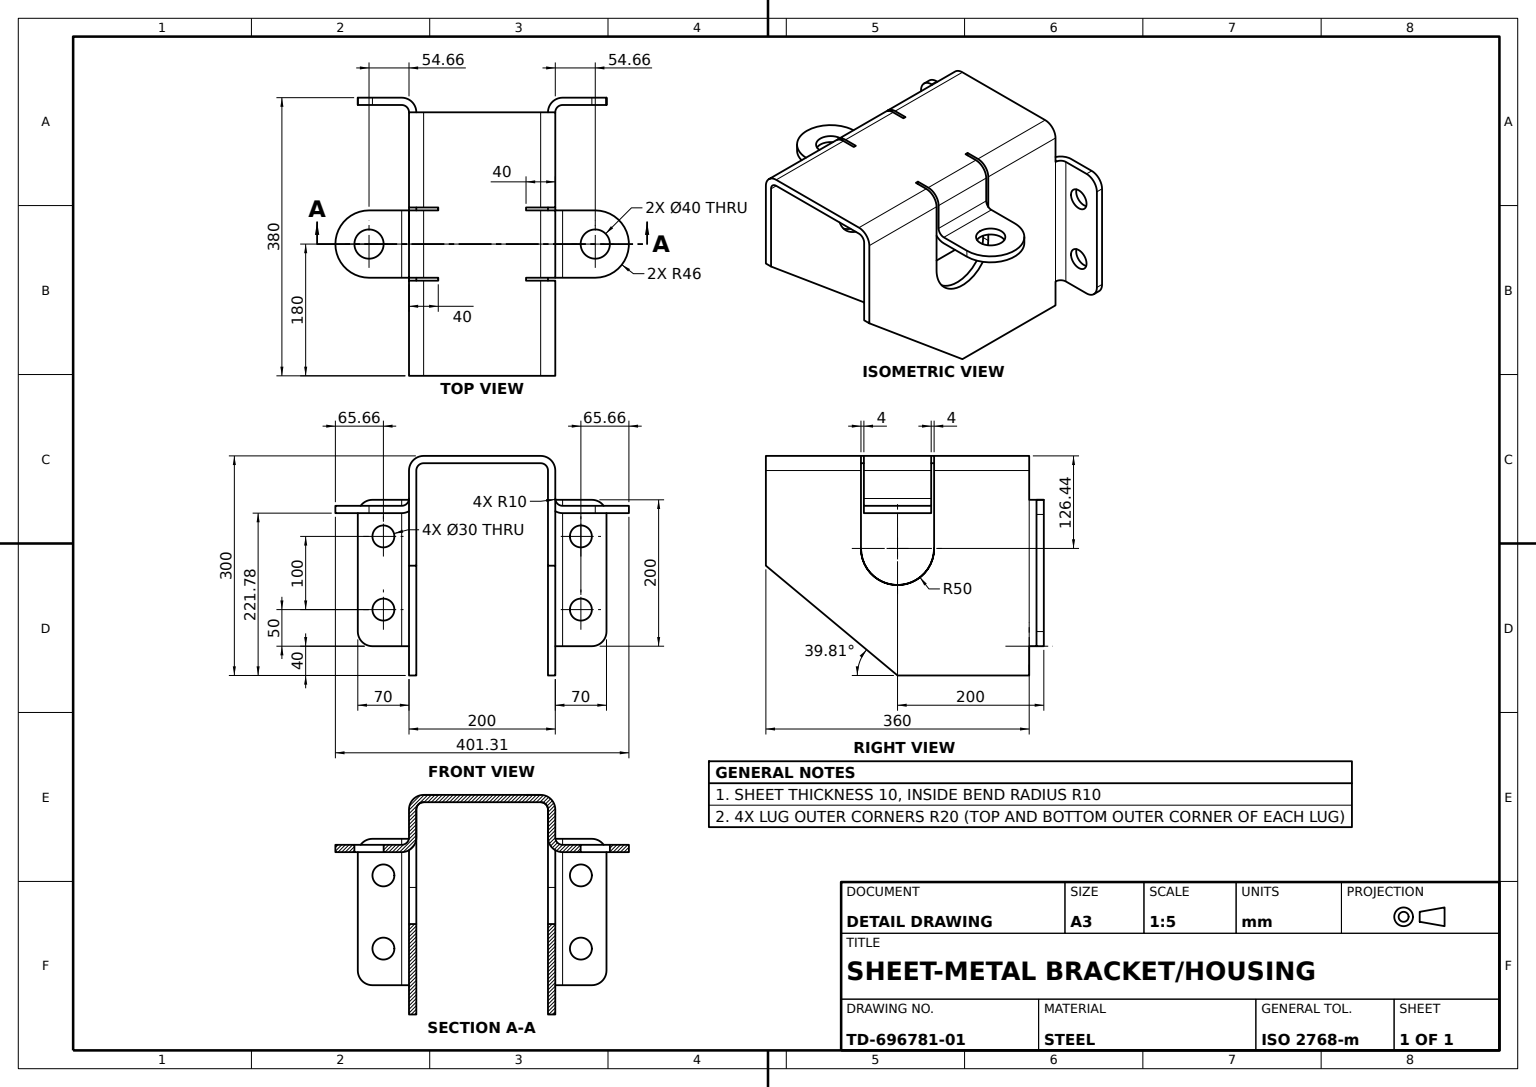
solid
v1 (0,-300,-100)
v2 (0,-300,-90)
e1 v1 v2 LINE
v3 (-180,-300,-90)
e2 v2 v3 LINE
v4 (-180,-300,-100)
e3 v4 v3 LINE
e4 v1 v4 LINE
face PLANE(AX(P(-180,-300,-100),D(0,1,0),D(0,0,1))) rev [e1 e2 -e3 -e4]
v5 (-46,0,-80)
v6 (-46,0,-60)
e5 v5 v6 LINE
v7 (-46,-10,-80)
e6 v7 v5 LINE
v8 (-46,-10,-60)
e7 v7 v8 LINE
e8 v8 v6 LINE
face PLANE(AX(P(-46,-10,-60),D(-1,0,0),D(0,0,1))) [-e5 -e6 e7 e8]
v9 (-46,-78.219028,110)
v10 (-46,-58.219028,90)
e9 v9 v10 CIRCLE(AX(P(-46,-58.219028,110),D(1,0,0),D(0,1,0)),20)
v11 (46,-58.219028,90)
e10 v11 v10 LINE
v12 (46,-78.219028,110)
e11 v11 v12 CIRCLE(AX(P(46,-58.219028,110),D(-1,0,0),D(0,-1,0)),20)
e12 v12 v9 LINE
face CYL(AX(P(95.49432,-58.219028,110),D(-1,0,0),D(0,-1,0)),20) [e9 -e10 e11 e12]
v13 (46,-68.219028,154.657083)
v14 (0,-68.219028,200.657083)
e13 v13 v14 CIRCLE(AX(P(0,-68.219028,154.657083),D(0,-1,0),D(0,0,1)),46)
v15 (0,-78.219028,200.657083)
e14 v15 v14 LINE
v16 (46,-78.219028,154.657083)
e15 v16 v15 CIRCLE(AX(P(0,-78.219028,154.657083),D(0,-1,0),D(0,0,1)),46)
e16 v16 v13 LINE
face CYL(AX(P(0,-78.219028,154.657083),D(0,1,0),D(0,0,1)),46) [e13 -e14 -e15 e16]
v17 (46,-20,-100)
v18 (46,0,-80)
e17 v17 v18 CIRCLE(AX(P(46,-20,-80),D(1,0,0),D(0,0,-1)),20)
v19 (-46,-20,-100)
e18 v19 v17 LINE
e19 v5 v19 CIRCLE(AX(P(-46,-20,-80),D(-1,0,0),D(0,0,-1)),20)
e20 v18 v5 LINE
face CYL(AX(P(-95.49432,-20,-80),D(1,0,0),D(0,0,-1)),20) [-e17 -e18 -e19 -e20]
v20 (-180,-300,100)
v21 (-180,-260,100)
e21 v20 v21 LINE
v22 (0,-300,100)
e22 v22 v20 LINE
v23 (180,-150,100)
e23 v23 v22 LINE
v24 (180,-20,100)
e24 v24 v23 LINE
v25 (50,-20,100)
e25 v24 v25 LINE
v26 (50,-126.438055,100)
e26 v26 v25 LINE
v27 (0,-176.438055,100)
e27 v27 v26 CIRCLE(AX(P(0,-126.438055,100),D(0,0,1),D(0,-1,0)),50)
v28 (-50,-126.438055,100)
e28 v28 v27 CIRCLE(AX(P(0,-126.438055,100),D(0,0,1),D(0,-1,0)),50)
v29 (-50,-20,100)
e29 v29 v28 LINE
v30 (-180,-20,100)
e30 v29 v30 LINE
v31 (-180,-60,100)
e31 v31 v30 LINE
e32 v21 v31 LINE
face PLANE(AX(P(0,0,100),D(0,0,1),D(0,-1,0))) [-e21 -e22 -e23 -e24 e25 -e26 -e27 -e28 -e29 e30 -e31 -e32]
v32 (-180,-60,-100)
v33 (-180,-20,-100)
e33 v32 v33 LINE
v34 (-50,-20,-100)
e34 v33 v34 LINE
v35 (-50,-126.438055,-100)
e35 v34 v35 LINE
v36 (50,-126.438055,-100)
e36 v35 v36 CIRCLE(AX(P(0,-126.438055,-100),D(0,0,1),D(0,-1,0)),50)
v37 (50,-20,-100)
e37 v36 v37 LINE
v38 (180,-20,-100)
e38 v37 v38 LINE
v39 (180,-150,-100)
e39 v38 v39 LINE
e40 v39 v1 LINE
v40 (-180,-260,-100)
e41 v4 v40 LINE
e42 v32 v40 LINE
face PLANE(AX(P(0,0,-100),D(0,0,-1),D(0,-1,0))) [e33 e34 e35 e36 e37 e38 e39 e40 e4 e41 -e42]
v41 (-200,-210,120)
v42 (-200,-210,150)
e43 v41 v42 CIRCLE(AX(P(-200,-210,135),D(-1,0,0),D(0,0,1)),15)
v43 (-190,-210,150)
e44 v42 v43 LINE
v44 (-190,-210,120)
e45 v44 v43 CIRCLE(AX(P(-190,-210,135),D(-1,0,0),D(0,0,1)),15)
e46 v41 v44 LINE
face CYL(AX(P(-200,-210,135),D(1,0,0),D(0,0,-1)),15) rev [e43 e44 -e45 -e46]
v45 (-46,-20,-90)
e47 v19 v45 LINE
e48 v7 v45 CIRCLE(AX(P(-46,-20,-80),D(-1,0,0),D(0,0,-1)),10)
face PLANE(AX(P(-46,-20,-80),D(1,0,0),D(0,0,-1))) rev [e6 e19 e47 -e48]
v46 (46,-20,-90)
v47 (46,-10,-80)
e49 v46 v47 CIRCLE(AX(P(46,-20,-80),D(1,0,0),D(0,0,1)),10)
e50 v47 v7 LINE
e51 v45 v46 LINE
face CYL(AX(P(-95.49432,-20,-80),D(1,0,0),D(0,0,-1)),10) rev [e49 e50 e48 e51]
v48 (46,-10,60)
v49 (46,-10,80)
e52 v48 v49 LINE
v50 (46,0,60)
e53 v48 v50 LINE
v51 (46,0,80)
e54 v50 v51 LINE
e55 v49 v51 LINE
face PLANE(AX(P(46,-10,60),D(-1,0,0),D(0,0,1))) rev [-e52 e53 e54 -e55]
v52 (-190,-60,110)
v53 (-190,-260,110)
e56 v52 v53 LINE
e57 v21 v53 CIRCLE(AX(P(-180,-260,110),D(0,1,0),D(0,0,1)),10)
e58 v52 v31 CIRCLE(AX(P(-180,-60,110),D(0,-1,0),D(0,0,1)),10)
face CYL(AX(P(-180,-361.631261,110),D(0,1,0),D(0,0,1)),10) rev [e56 -e57 e32 -e58]
v54 (46,-58.219028,-100)
e59 v17 v54 LINE
v55 (-46,-58.219028,-100)
e60 v55 v54 LINE
e61 v55 v19 LINE
face PLANE(AX(P(0,0,-100),D(0,0,-1),D(0,-1,0))) [e59 -e60 e61 e18]
v56 (50,-10,80)
v57 (180,-10,80)
e62 v56 v57 LINE
v58 (180,-20,90)
e63 v57 v58 CIRCLE(AX(P(180,-20,80),D(1,0,0),D(0,0,-1)),10)
v59 (50,-20,90)
e64 v58 v59 LINE
e65 v59 v56 CIRCLE(AX(P(50,-20,80),D(-1,0,0),D(0,0,1)),10)
face CYL(AX(P(247.495907,-20,80),D(-1,0,0),D(0,0,1)),10) rev [e62 e63 e64 e65]
v60 (46,-78.219028,-110)
v61 (46,-78.219028,-154.657083)
e66 v60 v61 LINE
v62 (46,-68.219028,-154.657083)
e67 v61 v62 LINE
v63 (46,-68.219028,-110)
e68 v63 v62 LINE
e69 v63 v60 LINE
face PLANE(AX(P(46,-78.219028,-4.657083),D(1,0,0),D(0,0,-1))) [e66 e67 -e68 e69]
v64 (46,-20,100)
e70 v51 v64 CIRCLE(AX(P(46,-20,80),D(1,0,0),D(0,0,1)),20)
v65 (46,-20,90)
e71 v64 v65 LINE
e72 v49 v65 CIRCLE(AX(P(46,-20,80),D(1,0,0),D(0,0,-1)),10)
face PLANE(AX(P(46,-20,80),D(-1,0,0),D(0,0,1))) rev [e70 e71 -e72 e55]
v66 (0,-78.219028,134.657083)
v67 (0,-68.219028,134.657083)
e73 v66 v67 LINE
v68 (0,-78.219028,174.657083)
e74 v68 v66 CIRCLE(AX(P(0,-78.219028,154.657083),D(0,1,0),D(0,0,1)),20)
v69 (0,-68.219028,174.657083)
e75 v68 v69 LINE
e76 v69 v67 CIRCLE(AX(P(0,-68.219028,154.657083),D(0,1,0),D(0,0,1)),20)
face CYL(AX(P(0,-78.219028,154.657083),D(0,1,0),D(0,0,1)),20) rev [-e73 -e74 e75 e76]
v70 (180,-150,90)
e77 v23 v70 LINE
e78 v58 v70 LINE
e79 v58 v24 LINE
face PLANE(AX(P(180,-150,100),D(1,0,0),D(0,1,0))) [e24 e77 -e78 e79]
v71 (180,-10,-80)
v72 (50,-10,-80)
e80 v71 v72 LINE
v73 (50,-20,-90)
e81 v72 v73 CIRCLE(AX(P(50,-20,-80),D(-1,0,0),D(0,0,-1)),10)
v74 (180,-20,-90)
e82 v73 v74 LINE
e83 v74 v71 CIRCLE(AX(P(180,-20,-80),D(1,0,0),D(0,0,-1)),10)
face CYL(AX(P(-17.495907,-20,-80),D(1,0,0),D(0,0,-1)),10) rev [e80 e81 e82 e83]
v75 (-200,-110,150)
v76 (-200,-110,120)
e84 v75 v76 CIRCLE(AX(P(-200,-110,135),D(-1,0,0),D(0,0,1)),15)
v77 (-190,-110,120)
e85 v76 v77 LINE
v78 (-190,-110,150)
e86 v78 v77 CIRCLE(AX(P(-190,-110,135),D(-1,0,0),D(0,0,1)),15)
e87 v75 v78 LINE
face CYL(AX(P(-200,-110,135),D(1,0,0),D(0,0,-1)),15) rev [e84 e85 -e86 -e87]
v79 (-50,-126.438055,-90)
e88 v79 v35 LINE
v80 (50,-126.438055,-90)
e89 v79 v80 CIRCLE(AX(P(0,-126.438055,-90),D(0,0,1),D(0,-1,0)),50)
e90 v80 v36 LINE
face CYL(AX(P(0,-126.438055,-90),D(0,0,-1),D(0,1,0)),50) rev [-e36 -e88 e89 e90]
v81 (-46,-78.219028,-154.657083)
e91 v61 v81 CIRCLE(AX(P(0,-78.219028,-154.657083),D(0,1,0),D(0,0,-1)),46)
v82 (-46,-68.219028,-154.657083)
e92 v81 v82 LINE
e93 v62 v82 CIRCLE(AX(P(0,-68.219028,-154.657083),D(0,1,0),D(0,0,-1)),46)
face CYL(AX(P(0,-78.219028,-154.657083),D(0,1,0),D(0,0,1)),46) [e91 e92 -e93 -e67]
v83 (0,-68.219028,-134.657083)
v84 (0,-68.219028,-174.657083)
e94 v83 v84 CIRCLE(AX(P(0,-68.219028,-154.657083),D(0,-1,0),D(0,0,-1)),20)
v85 (0,-78.219028,-134.657083)
e95 v85 v83 LINE
v86 (0,-78.219028,-174.657083)
e96 v85 v86 CIRCLE(AX(P(0,-78.219028,-154.657083),D(0,-1,0),D(0,0,-1)),20)
e97 v86 v84 LINE
face CYL(AX(P(0,-78.219028,-154.657083),D(0,1,0),D(0,0,1)),20) rev [-e94 -e95 e96 e97]
v87 (-200,-260,110)
e98 v53 v87 LINE
v88 (-190,-260,150)
e99 v53 v88 LINE
v89 (-200,-260,150)
e100 v89 v88 LINE
e101 v87 v89 LINE
face PLANE(AX(P(-200,-260,150),D(0,1,0),D(0,0,1))) rev [-e98 e99 -e100 -e101]
v90 (-46,-68.219028,-110)
e102 v55 v90 CIRCLE(AX(P(-46,-58.219028,-110),D(1,0,0),D(0,0,-1)),10)
v91 (-46,-78.219028,-110)
e103 v91 v90 LINE
v92 (-46,-58.219028,-90)
e104 v92 v91 CIRCLE(AX(P(-46,-58.219028,-110),D(1,0,0),D(0,0,-1)),20)
e105 v92 v55 LINE
face PLANE(AX(P(-46,-58.219028,-110),D(-1,0,0),D(0,0,1))) [e102 -e103 -e104 e105]
v93 (-180,-260,90)
v94 (-180,-60,90)
e106 v93 v94 LINE
e107 v93 v87 CIRCLE(AX(P(-180,-260,110),D(0,1,0),D(-1,0,0)),20)
v95 (-200,-60,110)
e108 v95 v87 LINE
e109 v95 v94 CIRCLE(AX(P(-180,-60,110),D(0,-1,0),D(0,0,-1)),20)
face CYL(AX(P(-180,-361.631261,110),D(0,1,0),D(0,0,1)),20) [-e106 e107 -e108 e109]
e110 v67 v69 CIRCLE(AX(P(0,-68.219028,154.657083),D(0,1,0),D(0,0,1)),20)
v96 (-46,-68.219028,154.657083)
e111 v14 v96 CIRCLE(AX(P(0,-68.219028,154.657083),D(0,-1,0),D(0,0,1)),46)
v97 (46,-68.219028,110)
e112 v97 v13 LINE
v98 (-46,-68.219028,110)
e113 v97 v98 LINE
e114 v96 v98 LINE
face PLANE(AX(P(0,-68.219028,28.219028),D(0,1,0),D(0,0,1))) [-e110 -e76] [-e111 -e13 -e112 e113 -e114]
v99 (-50,-10,-60)
e115 v8 v99 LINE
v100 (-50,0,-60)
e116 v99 v100 LINE
e117 v6 v100 LINE
face PLANE(AX(P(-50,-10,-60),D(0,0,-1),D(0,1,0))) [-e8 e115 e116 -e117]
v101 (-200,-80,170)
v102 (-200,-60,150)
e118 v101 v102 CIRCLE(AX(P(-200,-80,150),D(-1,0,0),D(0,0,1)),20)
v103 (-190,-80,170)
e119 v101 v103 LINE
v104 (-190,-60,150)
e120 v103 v104 CIRCLE(AX(P(-190,-80,150),D(-1,0,0),D(0,0,1)),20)
e121 v102 v104 LINE
face CYL(AX(P(-200,-80,150),D(1,0,0),D(0,0,-1)),20) [-e118 e119 e120 -e121]
v105 (-46,-78.219028,154.657083)
e122 v15 v105 CIRCLE(AX(P(0,-78.219028,154.657083),D(0,-1,0),D(0,0,1)),46)
e123 v105 v96 LINE
face CYL(AX(P(0,-78.219028,154.657083),D(0,1,0),D(0,0,1)),46) [-e122 e14 e111 -e123]
v106 (-46,-10,60)
v107 (-50,-10,60)
e124 v106 v107 LINE
v108 (-46,0,60)
e125 v106 v108 LINE
v109 (-50,0,60)
e126 v108 v109 LINE
e127 v107 v109 LINE
face PLANE(AX(P(-50,-10,60),D(0,0,-1),D(0,1,0))) rev [-e124 e125 e126 -e127]
v110 (-190,-260,-110)
e128 v110 v40 CIRCLE(AX(P(-180,-260,-110),D(0,1,0),D(0,0,-1)),10)
v111 (-190,-60,-110)
e129 v110 v111 LINE
e130 v32 v111 CIRCLE(AX(P(-180,-60,-110),D(0,-1,0),D(0,0,-1)),10)
face CYL(AX(P(-180,41.631261,-110),D(0,-1,0),D(0,0,-1)),10) rev [e42 -e128 e129 -e130]
v112 (-50,0,-80)
v113 (-50,-10,-80)
e131 v112 v113 LINE
e132 v100 v112 LINE
e133 v99 v113 LINE
face PLANE(AX(P(-50,-10,-60),D(1,0,0),D(0,0,-1))) [-e131 -e132 -e116 e133]
v114 (-180,0,80)
v115 (-50,0,80)
e134 v114 v115 LINE
e135 v109 v115 LINE
v116 (-46,0,80)
e136 v116 v108 LINE
e137 v116 v51 LINE
v117 (50,0,60)
e138 v117 v50 LINE
v118 (50,0,80)
e139 v118 v117 LINE
v119 (180,0,80)
e140 v118 v119 LINE
v120 (180,0,-80)
e141 v119 v120 LINE
v121 (50,0,-80)
e142 v120 v121 LINE
v122 (50,0,-60)
e143 v121 v122 LINE
v123 (46,0,-60)
e144 v122 v123 LINE
e145 v123 v18 LINE
v124 (-180,0,-80)
e146 v112 v124 LINE
e147 v124 v114 LINE
face PLANE(AX(P(0,0,0),D(0,-1,0),D(0,0,-1))) rev [e134 -e135 -e126 -e136 e137 -e54 -e138 -e139 e140 e141 e142 e143 e144 e145 e20 e5 e117 e132 e146 e147]
v125 (-190,-240,170)
e148 v88 v125 CIRCLE(AX(P(-190,-240,150),D(-1,0,0),D(0,0,1)),20)
v126 (-200,-240,170)
e149 v126 v125 LINE
e150 v89 v126 CIRCLE(AX(P(-200,-240,150),D(-1,0,0),D(0,0,1)),20)
face CYL(AX(P(-200,-240,150),D(1,0,0),D(0,0,-1)),20) [e100 e148 -e149 -e150]
v127 (-50,-20,90)
e151 v29 v127 LINE
v128 (-50,-10,80)
e152 v128 v127 CIRCLE(AX(P(-50,-20,80),D(1,0,0),D(0,0,-1)),10)
e153 v128 v115 LINE
e154 v115 v29 CIRCLE(AX(P(-50,-20,80),D(1,0,0),D(0,0,1)),20)
face PLANE(AX(P(-50,-20,80),D(-1,0,0),D(0,0,1))) rev [e151 -e152 e153 e154]
e155 v91 v60 LINE
v129 (46,-58.219028,-90)
e156 v60 v129 CIRCLE(AX(P(46,-58.219028,-110),D(-1,0,0),D(0,0,-1)),20)
e157 v92 v129 LINE
face CYL(AX(P(-95.49432,-58.219028,-110),D(1,0,0),D(0,0,-1)),20) [e155 e156 -e157 e104]
v130 (180,-150,-90)
e158 v130 v2 LINE
e159 v39 v130 LINE
face PLANE(AX(P(0,-300,-100),D(-0.6401844,0.76822128,0),D(-0.76822128,-0.6401844,0))) rev [e158 -e1 -e40 e159]
v131 (0,-176.438055,90)
e160 v131 v27 LINE
v132 (50,-126.438055,90)
e161 v132 v26 LINE
e162 v131 v132 CIRCLE(AX(P(0,-126.438055,90),D(0,0,1),D(0,-1,0)),50)
face CYL(AX(P(0,-126.438055,90),D(0,0,1),D(0,-1,0)),50) rev [e160 e27 -e161 -e162]
e163 v30 v114 CIRCLE(AX(P(-180,-20,80),D(-1,0,0),D(0,0,1)),20)
face CYL(AX(P(17.495907,-20,80),D(-1,0,0),D(0,0,1)),20) [-e163 -e30 -e154 -e134]
e164 v63 v54 CIRCLE(AX(P(46,-58.219028,-110),D(-1,0,0),D(0,0,-1)),10)
e165 v90 v63 LINE
face CYL(AX(P(-95.49432,-58.219028,-110),D(1,0,0),D(0,0,-1)),10) rev [e60 -e164 -e165 -e102]
e166 v84 v83 CIRCLE(AX(P(0,-68.219028,-154.657083),D(0,-1,0),D(0,0,-1)),20)
e167 v86 v85 CIRCLE(AX(P(0,-78.219028,-154.657083),D(0,-1,0),D(0,0,-1)),20)
face CYL(AX(P(0,-78.219028,-154.657083),D(0,1,0),D(0,0,1)),20) rev [-e166 -e97 e167 e95]
v133 (-200,-60,-110)
e168 v111 v133 LINE
v134 (-180,-60,-90)
e169 v134 v133 CIRCLE(AX(P(-180,-60,-110),D(0,-1,0),D(0,0,-1)),20)
e170 v32 v134 LINE
face PLANE(AX(P(-180,-60,-110),D(0,1,0),D(0,0,1))) [e168 -e169 -e170 e130]
e171 v65 v11 LINE
v135 (46,-58.219028,100)
e172 v64 v135 LINE
e173 v135 v11 LINE
face PLANE(AX(P(46,23.561945,90),D(-1,0,0),D(0,-1,0))) rev [-e171 -e71 e172 e173]
v136 (-46,-20,100)
e174 v64 v136 LINE
v137 (-46,-58.219028,100)
e175 v137 v136 LINE
e176 v135 v137 LINE
face PLANE(AX(P(0,0,100),D(0,0,1),D(0,-1,0))) [e174 -e175 -e176 -e172]
v138 (-180,-20,90)
e177 v94 v138 LINE
e178 v31 v94 LINE
e179 v138 v30 LINE
face PLANE(AX(P(-180,-10,100),D(-1,0,0),D(0,-1,0))) [-e177 -e178 e31 -e179]
v139 (-46,-20,90)
e180 v139 v136 LINE
e181 v10 v139 LINE
e182 v10 v137 LINE
face PLANE(AX(P(-46,23.561945,90),D(1,0,0),D(0,1,0))) rev [e175 -e180 -e181 e182]
e183 v54 v129 LINE
face PLANE(AX(P(46,-58.219028,-110),D(-1,0,0),D(0,0,1))) rev [-e69 e164 e183 -e156]
e184 v80 v73 LINE
e185 v37 v73 LINE
face PLANE(AX(P(50,23.561945,-90),D(-1,0,0),D(0,1,0))) [-e90 e184 -e185 -e37]
e186 v136 v116 CIRCLE(AX(P(-46,-20,80),D(-1,0,0),D(0,0,1)),20)
face CYL(AX(P(95.49432,-20,80),D(-1,0,0),D(0,0,1)),20) [-e174 -e70 -e137 -e186]
v140 (-180,-10,-80)
e187 v140 v124 LINE
v141 (-180,-10,80)
e188 v140 v141 LINE
e189 v141 v114 LINE
face PLANE(AX(P(-180,-10,100),D(-1,0,0),D(0,0,1))) [-e147 -e187 e188 e189]
e190 v66 v68 CIRCLE(AX(P(0,-78.219028,154.657083),D(0,1,0),D(0,0,1)),20)
face CYL(AX(P(0,-78.219028,154.657083),D(0,1,0),D(0,0,1)),20) rev [-e190 e73 e110 -e75]
v142 (-180,-20,-90)
e191 v140 v142 CIRCLE(AX(P(-180,-20,-80),D(-1,0,0),D(0,0,1)),10)
v143 (-50,-20,-90)
e192 v142 v143 LINE
e193 v143 v113 CIRCLE(AX(P(-50,-20,-80),D(1,0,0),D(0,0,1)),10)
e194 v113 v140 LINE
face CYL(AX(P(-247.495907,-20,-80),D(1,0,0),D(0,0,-1)),10) rev [e191 e192 e193 e194]
v144 (-180,-260,-90)
e195 v40 v144 LINE
e196 v3 v144 LINE
face PLANE(AX(P(-180,-10,-100),D(1,0,0),D(0,1,0))) rev [-e195 -e41 e3 e196]
v145 (-50,-126.438055,90)
e197 v145 v28 LINE
e198 v145 v131 CIRCLE(AX(P(0,-126.438055,90),D(0,0,1),D(0,-1,0)),50)
face CYL(AX(P(0,-126.438055,90),D(0,0,1),D(0,-1,0)),50) rev [e197 e28 -e160 -e198]
e199 v72 v121 LINE
e200 v121 v37 CIRCLE(AX(P(50,-20,-80),D(-1,0,0),D(0,0,-1)),20)
face PLANE(AX(P(50,-20,-80),D(1,0,0),D(0,0,-1))) rev [e199 e200 e185 -e81]
v146 (-200,-210,-120)
v147 (-190,-210,-120)
e201 v146 v147 LINE
v148 (-200,-210,-150)
e202 v148 v146 CIRCLE(AX(P(-200,-210,-135),D(1,0,0),D(0,0,1)),15)
v149 (-190,-210,-150)
e203 v148 v149 LINE
e204 v149 v147 CIRCLE(AX(P(-190,-210,-135),D(1,0,0),D(0,0,1)),15)
face CYL(AX(P(-200,-210,-135),D(1,0,0),D(0,0,-1)),15) rev [-e201 -e202 e203 e204]
e205 v92 v45 LINE
face PLANE(AX(P(-46,23.561945,-90),D(-1,0,0),D(0,1,0))) [-e47 -e61 -e105 e205]
e206 v57 v119 LINE
e207 v119 v24 CIRCLE(AX(P(180,-20,80),D(1,0,0),D(0,0,1)),20)
face PLANE(AX(P(180,-20,80),D(-1,0,0),D(0,0,1))) rev [e206 e207 -e79 -e63]
e208 v146 v148 CIRCLE(AX(P(-200,-210,-135),D(1,0,0),D(0,0,1)),15)
e209 v147 v149 CIRCLE(AX(P(-190,-210,-135),D(1,0,0),D(0,0,1)),15)
face CYL(AX(P(-200,-210,-135),D(1,0,0),D(0,0,-1)),15) rev [-e203 -e208 e201 e209]
v150 (-200,-110,-120)
v151 (-200,-110,-150)
e210 v150 v151 CIRCLE(AX(P(-200,-110,-135),D(1,0,0),D(0,0,1)),15)
e211 v151 v150 CIRCLE(AX(P(-200,-110,-135),D(1,0,0),D(0,0,1)),15)
v152 (-200,-260,-110)
v153 (-200,-260,-150)
e212 v152 v153 LINE
e213 v152 v133 LINE
v154 (-200,-60,-150)
e214 v154 v133 LINE
v155 (-200,-80,-170)
e215 v155 v154 CIRCLE(AX(P(-200,-80,-150),D(1,0,0),D(0,0,1)),20)
v156 (-200,-240,-170)
e216 v156 v155 LINE
e217 v153 v156 CIRCLE(AX(P(-200,-240,-150),D(1,0,0),D(0,0,1)),20)
face PLANE(AX(P(-200,-80,-150),D(-1,0,0),D(0,0,-1))) [e210 e211] [-e212 e213 -e214 -e215 -e216 -e217] [e208 e202]
v157 (-190,-110,-150)
v158 (-190,-110,-120)
e218 v157 v158 CIRCLE(AX(P(-190,-110,-135),D(1,0,0),D(0,0,1)),15)
e219 v158 v157 CIRCLE(AX(P(-190,-110,-135),D(1,0,0),D(0,0,1)),15)
v159 (-190,-240,-170)
v160 (-190,-80,-170)
e220 v159 v160 LINE
v161 (-190,-60,-150)
e221 v160 v161 CIRCLE(AX(P(-190,-80,-150),D(1,0,0),D(0,0,1)),20)
e222 v161 v111 LINE
v162 (-190,-260,-150)
e223 v110 v162 LINE
e224 v162 v159 CIRCLE(AX(P(-190,-240,-150),D(1,0,0),D(0,0,1)),20)
face PLANE(AX(P(-190,-80,-150),D(-1,0,0),D(0,0,-1))) rev [-e218 -e219] [-e209 -e204] [e220 e221 e222 -e129 e223 e224]
e225 v82 v90 LINE
face PLANE(AX(P(0,-68.219028,-28.219028),D(0,1,0),D(0,0,-1))) [e93 e225 e165 e68] [e166 e94]
e226 v135 v97 CIRCLE(AX(P(46,-58.219028,110),D(-1,0,0),D(0,-1,0)),10)
e227 v97 v12 LINE
face PLANE(AX(P(46,-58.219028,110),D(1,0,0),D(0,1,0))) [-e11 -e173 e226 e227]
e228 v132 v59 LINE
e229 v59 v25 LINE
face PLANE(AX(P(50,23.561945,90),D(1,0,0),D(0,1,0))) rev [-e228 e161 e26 -e229]
v163 (-46,-10,80)
e230 v139 v163 CIRCLE(AX(P(-46,-20,80),D(-1,0,0),D(0,0,1)),10)
e231 v116 v163 LINE
face PLANE(AX(P(-46,-20,80),D(1,0,0),D(0,0,-1))) rev [-e230 e180 e186 e231]
v164 (50,-10,-60)
e232 v72 v164 LINE
e233 v164 v122 LINE
face PLANE(AX(P(50,-10,-60),D(-1,0,0),D(0,0,1))) [e232 e233 -e143 -e199]
e234 v43 v44 CIRCLE(AX(P(-190,-210,135),D(-1,0,0),D(0,0,1)),15)
e235 v42 v41 CIRCLE(AX(P(-200,-210,135),D(-1,0,0),D(0,0,1)),15)
face CYL(AX(P(-200,-210,135),D(1,0,0),D(0,0,-1)),15) rev [-e234 -e44 e235 e46]
v165 (0,-300,90)
v166 (-180,-300,90)
e236 v165 v166 LINE
e237 v22 v165 LINE
e238 v20 v166 LINE
face PLANE(AX(P(-180,-300,100),D(0,-1,0),D(0,0,-1))) [-e236 -e237 e22 e238]
e239 v70 v165 LINE
face PLANE(AX(P(0,-300,100),D(0.6401844,-0.76822128,0),D(0.76822128,0.6401844,0))) [e23 e237 -e239 -e77]
e240 v81 v91 LINE
face PLANE(AX(P(0,-78.219028,-28.219028),D(0,1,0),D(0,0,-1))) rev [-e240 -e91 -e66 -e155] [-e96 -e167]
e241 v110 v152 LINE
e242 v152 v144 CIRCLE(AX(P(-180,-260,-110),D(0,1,0),D(0,0,1)),20)
face PLANE(AX(P(-180,-260,-110),D(0,-1,0),D(0,0,-1))) [-e241 e128 e195 -e242]
e243 v25 v118 CIRCLE(AX(P(50,-20,80),D(-1,0,0),D(0,0,1)),20)
e244 v118 v56 LINE
face PLANE(AX(P(50,-20,80),D(1,0,0),D(0,0,-1))) rev [-e65 e229 e243 e244]
e245 v46 v17 LINE
e246 v46 v129 LINE
face PLANE(AX(P(46,23.561945,-90),D(1,0,0),D(0,-1,0))) [-e183 -e59 -e245 e246]
e247 v38 v120 CIRCLE(AX(P(180,-20,-80),D(1,0,0),D(0,0,-1)),20)
face CYL(AX(P(-17.495907,-20,-80),D(1,0,0),D(0,0,-1)),20) [-e38 -e200 -e142 -e247]
face CYL(AX(P(247.495907,-20,80),D(-1,0,0),D(0,0,1)),20) [-e25 -e207 -e140 -e243]
e248 v74 v38 LINE
e249 v74 v130 LINE
face PLANE(AX(P(180,-150,-100),D(-1,0,0),D(0,-1,0))) rev [-e39 -e248 e249 -e159]
v167 (50,-10,60)
e250 v167 v117 LINE
e251 v56 v167 LINE
face PLANE(AX(P(50,-10,60),D(1,0,0),D(0,0,-1))) rev [-e244 e139 -e250 -e251]
e252 v105 v9 LINE
e253 v12 v16 LINE
face PLANE(AX(P(0,-78.219028,28.219028),D(0,1,0),D(0,0,1))) rev [e190 e74] [e15 e122 e252 -e12 e253]
e254 v71 v120 LINE
face PLANE(AX(P(180,-20,-80),D(-1,0,0),D(0,0,1))) rev [e248 e247 -e254 -e83]
e255 v52 v95 LINE
e256 v102 v95 LINE
e257 v104 v52 LINE
face PLANE(AX(P(-200,-60,100),D(0,-1,0),D(0,0,-1))) rev [e255 -e256 e121 e257]
e258 v98 v137 CIRCLE(AX(P(-46,-58.219028,110),D(1,0,0),D(0,-1,0)),10)
face CYL(AX(P(95.49432,-58.219028,110),D(-1,0,0),D(0,-1,0)),10) rev [-e258 -e113 -e226 e176]
e259 v21 v93 LINE
e260 v166 v93 LINE
face PLANE(AX(P(-180,-10,100),D(-1,0,0),D(0,-1,0))) [e21 e259 -e260 -e238]
e261 v126 v101 LINE
e262 v76 v75 CIRCLE(AX(P(-200,-110,135),D(-1,0,0),D(0,0,1)),15)
face PLANE(AX(P(-200,-80,150),D(-1,0,0),D(0,0,1))) [e101 e150 e261 e118 e256 e108] [-e84 -e262] [-e235 -e43]
v168 (46,-10,-60)
e263 v168 v47 LINE
e264 v164 v168 LINE
e265 v57 v71 LINE
e266 v167 v48 LINE
e267 v163 v49 LINE
e268 v163 v106 LINE
e269 v107 v128 LINE
e270 v141 v128 LINE
face PLANE(AX(P(0,-10,0),D(0,-1,0),D(0,0,-1))) [-e7 -e50 -e263 -e264 -e232 -e80 -e265 -e62 e251 e266 e52 -e267 e268 e124 e269 -e270 -e188 -e194 -e133 -e115]
face PLANE(AX(P(50,-10,60),D(0,0,-1),D(0,1,0))) rev [e250 e138 -e53 -e266]
e271 v155 v160 LINE
e272 v154 v161 LINE
face CYL(AX(P(-200,-80,-150),D(1,0,0),D(0,0,-1)),20) [-e221 -e271 e215 e272]
e273 v18 v47 LINE
e274 v168 v123 LINE
face PLANE(AX(P(46,-10,-60),D(1,0,0),D(0,0,-1))) [-e273 -e145 -e274 e263]
e275 v153 v162 LINE
face PLANE(AX(P(-200,-260,-150),D(0,-1,0),D(0,0,-1))) [e241 e212 e275 -e223]
e276 v65 v139 LINE
face PLANE(AX(P(0,0,90),D(0,0,1),D(0,-1,0))) rev [e181 -e276 e171 e10]
face PLANE(AX(P(46,-20,-80),D(-1,0,0),D(0,0,1))) rev [e245 e17 e273 -e49]
face PLANE(AX(P(50,-10,-60),D(0,0,-1),D(0,1,0))) [e274 -e144 -e233 e264]
e277 v142 v33 LINE
e278 v134 v142 LINE
face PLANE(AX(P(-180,-10,-100),D(1,0,0),D(0,1,0))) rev [e277 -e33 e170 e278]
e279 v143 v79 LINE
e280 v134 v144 LINE
face PLANE(AX(P(0,0,-90),D(0,0,-1),D(0,-1,0))) rev [-e2 -e158 -e249 -e82 -e184 -e89 -e279 -e192 -e278 e280 -e196]
e281 v156 v159 LINE
face PLANE(AX(P(-200,-80,-170),D(0,0,-1),D(-1,0,0))) [-e281 e216 e271 -e220]
face PLANE(AX(P(0,0,-90),D(0,0,-1),D(0,-1,0))) rev [-e205 e157 -e246 -e51]
face PLANE(AX(P(-200,-60,-100),D(0,1,0),D(0,0,1))) [e214 -e168 -e222 -e272]
e282 v127 v145 LINE
face PLANE(AX(P(-50,23.561945,90),D(-1,0,0),D(0,-1,0))) rev [-e282 -e151 e29 -e197]
e283 v143 v34 LINE
e284 v34 v112 CIRCLE(AX(P(-50,-20,-80),D(1,0,0),D(0,0,-1)),20)
face PLANE(AX(P(-50,-20,-80),D(-1,0,0),D(0,0,1))) rev [e283 e284 e131 -e193]
face CYL(AX(P(-180,41.631261,-110),D(0,-1,0),D(0,0,-1)),20) [-e280 e169 -e213 e242]
face PLANE(AX(P(-46,-78.219028,-4.657083),D(-1,0,0),D(0,0,1))) [e240 e103 -e225 -e92]
face PLANE(AX(P(-50,23.561945,-90),D(1,0,0),D(0,-1,0))) [-e283 e279 e88 -e35]
e285 v151 v157 LINE
e286 v150 v158 LINE
face CYL(AX(P(-200,-110,-135),D(1,0,0),D(0,0,-1)),15) rev [e219 -e285 -e210 e286]
e287 v138 v141 CIRCLE(AX(P(-180,-20,80),D(-1,0,0),D(0,-1,0)),10)
face PLANE(AX(P(-180,-20,80),D(1,0,0),D(0,1,0))) rev [e179 e163 -e189 -e287]
e288 v125 v103 LINE
e289 v77 v78 CIRCLE(AX(P(-190,-110,135),D(-1,0,0),D(0,0,1)),15)
face PLANE(AX(P(-190,-80,150),D(-1,0,0),D(0,0,1))) rev [-e56 -e257 -e120 -e288 -e148 -e99] [e234 e45] [e289 e86]
face CYL(AX(P(-200,-110,135),D(1,0,0),D(0,0,-1)),15) rev [e262 e87 -e289 -e85]
face PLANE(AX(P(-50,-10,60),D(-1,0,0),D(0,0,1))) rev [-e153 -e269 e127 e135]
face CYL(AX(P(95.49432,-20,80),D(-1,0,0),D(0,0,1)),10) rev [e267 e72 e276 e230]
e290 v9 v98 LINE
face PLANE(AX(P(-46,-78.219028,4.657083),D(1,0,0),D(0,0,-1))) rev [e114 -e290 -e252 e123]
e291 v127 v138 LINE
face PLANE(AX(P(0,0,90),D(0,0,1),D(0,-1,0))) rev [e162 e228 -e64 e78 e239 e236 e260 e106 e177 -e291 e282 e198]
face PLANE(AX(P(-180,-260,110),D(0,-1,0),D(1,0,0))) [-e107 -e259 e57 e98]
face PLANE(AX(P(-46,-10,60),D(1,0,0),D(0,0,-1))) rev [-e125 -e268 -e231 e136]
face PLANE(AX(P(46,-78.219028,4.657083),D(-1,0,0),D(0,0,1))) rev [e112 -e16 -e253 -e227]
face PLANE(AX(P(-200,-80,170),D(0,0,-1),D(-1,0,0))) rev [e288 -e119 -e261 e149]
face CYL(AX(P(-200,-240,-150),D(1,0,0),D(0,0,-1)),20) [-e275 e217 e281 -e224]
face PLANE(AX(P(180,-10,100),D(1,0,0),D(0,0,-1))) [e265 e254 -e141 -e206]
e292 v124 v33 CIRCLE(AX(P(-180,-20,-80),D(-1,0,0),D(0,0,-1)),20)
face PLANE(AX(P(-180,-20,-80),D(1,0,0),D(0,0,-1))) rev [-e277 -e191 e187 e292]
face PLANE(AX(P(-46,-58.219028,110),D(-1,0,0),D(0,-1,0))) [-e182 -e9 e290 e258]
face PLANE(AX(P(-180,-60,110),D(0,1,0),D(0,0,1))) [e178 -e109 -e255 e58]
face CYL(AX(P(17.495907,-20,80),D(-1,0,0),D(0,0,1)),10) rev [e152 e291 e287 e270]
face CYL(AX(P(-200,-110,-135),D(1,0,0),D(0,0,-1)),15) rev [e218 -e286 -e211 e285]
face CYL(AX(P(-247.495907,-20,-80),D(1,0,0),D(0,0,-1)),20) [-e292 -e146 -e284 -e34]
